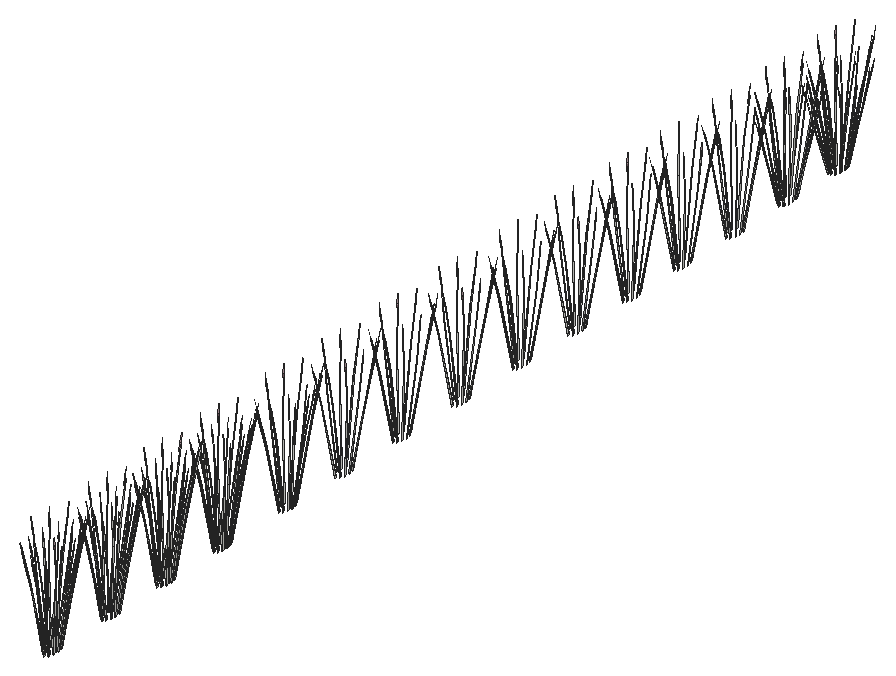
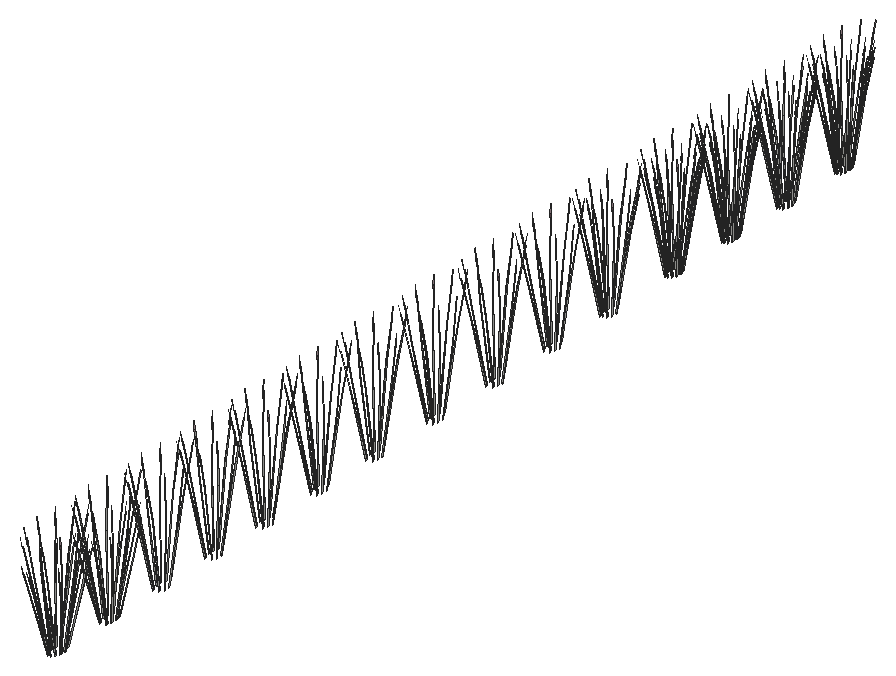
# SketchUp Ruby script. Lengths in inches.
U = 1.inch
M = Sketchup.active_model
def pt(a) = Geom::Point3d.new(a.map { |v| v * U })
def face(e, loops, mat)
  f = e.add_face(loops[0].map { |a| pt(a) })
  loops[1..].each { |l| e.add_face(l.map { |a| pt(a) }).erase! }
  f.material = f.back_material = mat if mat
  f
end
# faces: each face lists its corners as indices into pts; further lists are holes
def faces(e, pts, list, mat = nil) = list.each { |f| face(e, (f[0].is_a?(Array) ? f : [f]).map { |l| l.map { |i| pts[i] } }, mat) }
# xy, xz, yz: faces in a plane at the given z, y or x. An outline is a flat list of corners, or four numbers for a rectangle; further outlines are holes
def ring(l) = l.size == 4 ? [[l[0], l[1]], [l[2], l[1]], [l[2], l[3]], [l[0], l[3]]] : l.each_slice(2).to_a
def flat(e, list, mat, &to3) = list.each { |f| face(e, (f[0].is_a?(Array) ? f : [f]).map { |l| ring(l).map { |u, v| to3.(u, v) } }, mat) }
def xy(e, z, list, mat = nil) = flat(e, list, mat) { |x, y| [x, y, z] }
def xz(e, y, list, mat = nil) = flat(e, list, mat) { |x, z| [x, y, z] }
def yz(e, x, list, mat = nil) = flat(e, list, mat) { |y, z| [x, y, z] }
def lines(e, pts, list) = list.each { |a, b| e.add_line(pt(pts[a]), pt(pts[b])) }
# prism: a flat outline (further loops are holes) pulled along v
def prism(e, loops, v, mat = nil)
  f = face(e, loops, mat); d = Geom::Vector3d.new(v.map { |x| x * U })
  f.pushpull(f.normal.samedirection?(d) ? d.length : -d.length)
end
def box(e, o, s, mat = nil) = prism(e, [[o, [o[0] + s[0], o[1], o[2]], [o[0] + s[0], o[1] + s[1], o[2]], [o[0], o[1] + s[1], o[2]]]], [0, 0, s[2]], mat)
def at(x, y, z, deg = 0) = Geom::Transformation.translation(pt([x, y, z])) * Geom::Transformation.rotation(ORIGIN, Z_AXIS, deg.degrees)
def axes(o, x, y, z) = Geom::Transformation.new([*x, 0, *y, 0, *z, 0, *pt(o).to_a, 1])
def part(name) = M.definitions.add(name)
# library, detail: a bought-in or finely detailed component or shape, given as its bounding box
def library(name, o, s) = part(name).tap { |d| box(d.entities, o, s) }
def detail(e, o, s) = box(e.add_group.entities, o, s)
def put(e, d, t, mat = nil) = e.add_instance(d, t).tap { |i| i.material = mat if mat }
def group(e, t, mat = nil) = e.add_group.tap { |g| g.transformation = t; g.material = mat if mat }.entities
root = M.entities
M.materials.add("LightPink_Translucent").color = [144, 107, 117]
M.materials["LightPink_Translucent"].alpha = 0.75
c1 = part("blade")
p = [[2.15,0.21,22],[0,0.17,0],[0.09,0.45,0],[2.18,0.31,22],[2.29,0.31,22],[0.38,0.45,0],
  [2.48,0.24,33],[2.49,0.24,33],[2.48,0.22,33]]
faces(c1.entities,p,[[0,1,2,3],[4,5,2,3],[6,3,4,7],[8,0,3,6]])
c2 = part("seeds")
p = [[0.3,-0.1,1.38],[-0.01,-0.03,1.59],[-0.01,-0.03,0.03],[0.14,-0.07,-0.07],[0.29,-0.03,3],[0.15,0.01,3.11]]
faces(c2.entities,p,[[0,1,2,3],[1,0,4,5]],"LightPink_Translucent")
c3 = part("blade with seeds")
put(c3.entities,c1,at(0,0,0))
put(c3.entities,c2,axes([2.4,0.25,30.99],[1.5799,-0.05474,1.17369],[-0.12525,1.92788,0.29478],[-0.07173,-0.02425,1.56792]))
put(root,c3,axes([250.75,226.01,2.625],[0.01289,-0.46496,0.04667],[0.19462,0.01275,0.3674],[-0.07455,-0.04865,0.56022]))
put(root,c3,axes([252.51,225.85,2.625],[0.21034,0.02849,0.04667],[-0.00577,0.43021,0.3674],[0.02201,-0.1648,0.56022]))
put(root,c3,axes([252.58,229.75,2.625],[-0.01289,0.46496,0.04667],[-0.19462,-0.01275,0.3674],[0.07455,0.04865,0.56022]))
put(root,c3,axes([250.47,228.7,2.625],[-0.17571,-0.25715,0.04667],[0.1023,-0.3662,0.3674],[-0.05634,0.11839,0.56022]))
put(root,c3,axes([251.9375,225.18,2.625],[0.1886,-0.20781,0.04667],[0.09231,0.37894,0.3674],[-0.01821,-0.16704,0.56022]))
put(root,c3,axes([250.44,227.27,2.625],[-0.09401,-0.41691,0.04667],[0.17143,-0.20406,0.3674],[-0.07557,0.04026,0.56022]))
put(root,c3,axes([252.04,230.51,2.625],[-0.11633,0.38842,0.04667],[-0.16566,-0.22614,0.3674],[0.05356,0.12453,0.56022]))
put(root,c3,axes([250.82,229.91,2.625],[-0.21034,-0.02849,0.04667],[0.00577,-0.43021,0.3674],[-0.02201,0.1648,0.56022]))
put(root,c3,axes([251.29,240.33,2.625],[0.11633,-0.38842,0.04667],[0.16566,0.22614,0.3674],[-0.05356,-0.12453,0.56022]))
put(root,c3,axes([251.39,245.66,2.625],[-0.1886,0.20781,0.04667],[-0.09231,-0.37894,0.3674],[0.01821,0.16704,0.56022]))
put(root,c3,axes([252.86,242.14,2.625],[0.17571,0.25715,0.04667],[-0.1023,0.3662,0.3674],[0.05634,-0.11839,0.56022]))
put(root,c3,axes([252.88,243.57,2.625],[0.09401,0.41691,0.04667],[-0.17143,0.20406,0.3674],[0.07557,-0.04026,0.56022]))
put(root,c3,axes([250.75,241.09,2.625],[0.01289,-0.46496,0.04667],[0.19462,0.01275,0.3674],[-0.07455,-0.04865,0.56022]))
put(root,c3,axes([252.51,240.93,2.625],[0.21034,0.02849,0.04667],[-0.00577,0.43021,0.3674],[0.02201,-0.1648,0.56022]))
put(root,c3,axes([252.58,244.83,2.625],[-0.01289,0.46496,0.04667],[-0.19462,-0.01275,0.3674],[0.07455,0.04865,0.56022]))
put(root,c3,axes([250.47,243.78,2.625],[-0.17571,-0.25715,0.04667],[0.1023,-0.3662,0.3674],[-0.05634,0.11839,0.56022]))
put(root,c3,axes([251.9375,240.27,2.625],[0.1886,-0.20781,0.04667],[0.09231,0.37894,0.3674],[-0.01821,-0.16704,0.56022]))
put(root,c3,axes([250.44,242.36,2.625],[-0.09401,-0.41691,0.04667],[0.17143,-0.20406,0.3674],[-0.07557,0.04026,0.56022]))
put(root,c3,axes([252.04,245.6,2.625],[-0.11633,0.38842,0.04667],[-0.16566,-0.22614,0.3674],[0.05356,0.12453,0.56022]))
put(root,c3,axes([250.82,244.99,2.625],[-0.21034,-0.02849,0.04667],[0.00577,-0.43021,0.3674],[-0.02201,0.1648,0.56022]))
put(root,c3,axes([251.87,10.4375,2.63],[0.25221,0.15985,0.34839],[-0.08624,0.52553,0.28727],[-0.01516,-0.20667,0.72092]))
put(root,c3,axes([252.6,14.82,2.63],[-0.18873,0.4029,0.34839],[-0.16277,-0.42787,0.28727],[0.08855,0.07432,0.72092]))
put(root,c3,axes([252.86,13.55,2.63],[-0.07231,0.55752,0.34839],[-0.23774,-0.19064,0.28727],[0.09349,-0.0335,0.72092]))
put(root,c3,axes([250.52,14.02,2.63],[-0.06348,-0.56275,0.34839],[0.24901,-0.09767,0.28727],[-0.07339,0.13235,0.72092]))
put(root,c3,axes([250.88,15.16,2.63],[-0.18226,-0.41719,0.34839],[0.19356,-0.3598,0.28727],[-0.03362,0.19573,0.72092]))
put(root,c3,axes([252.44,11.02,2.63],[0.18226,0.41719,0.34839],[-0.19356,0.3598,0.28727],[0.03362,-0.19573,0.72092]))
put(root,c3,axes([250.46,12.63,2.63],[0.07231,-0.55752,0.34839],[0.23774,0.19064,0.28727],[-0.09349,0.0335,0.72092]))
put(root,c3,axes([252.81,12.16,2.63],[0.06348,0.56275,0.34839],[-0.24901,0.09767,0.28727],[0.07339,-0.13235,0.72092]))
put(root,c3,axes([252.08,15.62,2.63],[-0.25458,0.14032,0.34839],[-0.04418,-0.55045,0.28727],[0.05987,0.16223,0.72092]))
put(root,c3,axes([251.87,27.31,2.63],[0.25221,0.15985,0.34839],[-0.08624,0.52553,0.28727],[-0.01516,-0.20667,0.72092]))
put(root,c3,axes([252.6,31.68,2.63],[-0.18873,0.4029,0.34839],[-0.16277,-0.42787,0.28727],[0.08855,0.07432,0.72092]))
put(root,c3,axes([252.86,30.42,2.63],[-0.07231,0.55752,0.34839],[-0.23774,-0.19064,0.28727],[0.09349,-0.0335,0.72092]))
put(root,c3,axes([250.52,30.89,2.63],[-0.06348,-0.56275,0.34839],[0.24901,-0.09767,0.28727],[-0.07339,0.13235,0.72092]))
put(root,c3,axes([250.88,32.03,2.63],[-0.18226,-0.41719,0.34839],[0.19356,-0.3598,0.28727],[-0.03362,0.19573,0.72092]))
put(root,c3,axes([252.44,27.89,2.63],[0.18226,0.41719,0.34839],[-0.19356,0.3598,0.28727],[0.03362,-0.19573,0.72092]))
put(root,c3,axes([250.46,29.5,2.63],[0.07231,-0.55752,0.34839],[0.23774,0.19064,0.28727],[-0.09349,0.0335,0.72092]))
put(root,c3,axes([252.81,29.03,2.63],[0.06348,0.56275,0.34839],[-0.24901,0.09767,0.28727],[0.07339,-0.13235,0.72092]))
put(root,c3,axes([252.08,32.49,2.63],[-0.25458,0.14032,0.34839],[-0.04418,-0.55045,0.28727],[0.05987,0.16223,0.72092]))
put(root,c3,axes([251.87,43.46,2.63],[0.25221,0.15985,0.34839],[-0.08624,0.52553,0.28727],[-0.01516,-0.20667,0.72092]))
put(root,c3,axes([252.6,47.84,2.63],[-0.18873,0.4029,0.34839],[-0.16277,-0.42787,0.28727],[0.08855,0.07432,0.72092]))
put(root,c3,axes([252.86,46.57,2.63],[-0.07231,0.55752,0.34839],[-0.23774,-0.19064,0.28727],[0.09349,-0.0335,0.72092]))
put(root,c3,axes([250.52,47.04,2.63],[-0.06348,-0.56275,0.34839],[0.24901,-0.09767,0.28727],[-0.07339,0.13235,0.72092]))
put(root,c3,axes([250.88,48.18,2.63],[-0.18226,-0.41719,0.34839],[0.19356,-0.3598,0.28727],[-0.03362,0.19573,0.72092]))
put(root,c3,axes([252.44,44.04,2.63],[0.18226,0.41719,0.34839],[-0.19356,0.3598,0.28727],[0.03362,-0.19573,0.72092]))
put(root,c3,axes([250.46,45.65,2.63],[0.07231,-0.55752,0.34839],[0.23774,0.19064,0.28727],[-0.09349,0.0335,0.72092]))
put(root,c3,axes([252.81,45.18,2.63],[0.06348,0.56275,0.34839],[-0.24901,0.09767,0.28727],[0.07339,-0.13235,0.72092]))
put(root,c3,axes([252.08,48.64,2.63],[-0.25458,0.14032,0.34839],[-0.04418,-0.55045,0.28727],[0.05987,0.16223,0.72092]))
put(root,c3,axes([251.87,59.91,2.63],[0.25221,0.15985,0.34839],[-0.08624,0.52553,0.28727],[-0.01516,-0.20667,0.72092]))
put(root,c3,axes([252.6,64.29,2.63],[-0.18873,0.4029,0.34839],[-0.16277,-0.42787,0.28727],[0.08855,0.07432,0.72092]))
put(root,c3,axes([252.86,63.02,2.63],[-0.07231,0.55752,0.34839],[-0.23774,-0.19064,0.28727],[0.09349,-0.0335,0.72092]))
put(root,c3,axes([250.52,63.49,2.63],[-0.06348,-0.56275,0.34839],[0.24901,-0.09767,0.28727],[-0.07339,0.13235,0.72092]))
put(root,c3,axes([250.88,64.63,2.63],[-0.18226,-0.41719,0.34839],[0.19356,-0.3598,0.28727],[-0.03362,0.19573,0.72092]))
put(root,c3,axes([252.44,60.49,2.63],[0.18226,0.41719,0.34839],[-0.19356,0.3598,0.28727],[0.03362,-0.19573,0.72092]))
put(root,c3,axes([250.46,62.1,2.63],[0.07231,-0.55752,0.34839],[0.23774,0.19064,0.28727],[-0.09349,0.0335,0.72092]))
put(root,c3,axes([252.81,61.63,2.63],[0.06348,0.56275,0.34839],[-0.24901,0.09767,0.28727],[0.07339,-0.13235,0.72092]))
put(root,c3,axes([252.08,65.09,2.63],[-0.25458,0.14032,0.34839],[-0.04418,-0.55045,0.28727],[0.05987,0.16223,0.72092]))
put(root,c3,axes([251.87,78.93,2.63],[0.25221,0.15985,0.34839],[-0.08624,0.52553,0.28727],[-0.01516,-0.20667,0.72092]))
put(root,c3,axes([252.6,83.3125,2.63],[-0.18873,0.4029,0.34839],[-0.16277,-0.42787,0.28727],[0.08855,0.07432,0.72092]))
put(root,c3,axes([252.86,82.04,2.63],[-0.07231,0.55752,0.34839],[-0.23774,-0.19064,0.28727],[0.09349,-0.0335,0.72092]))
put(root,c3,axes([250.52,82.52,2.63],[-0.06348,-0.56275,0.34839],[0.24901,-0.09767,0.28727],[-0.07339,0.13235,0.72092]))
put(root,c3,axes([250.88,83.66,2.63],[-0.18226,-0.41719,0.34839],[0.19356,-0.3598,0.28727],[-0.03362,0.19573,0.72092]))
put(root,c3,axes([252.44,79.52,2.63],[0.18226,0.41719,0.34839],[-0.19356,0.3598,0.28727],[0.03362,-0.19573,0.72092]))
put(root,c3,axes([250.46,81.13,2.63],[0.07231,-0.55752,0.34839],[0.23774,0.19064,0.28727],[-0.09349,0.0335,0.72092]))
put(root,c3,axes([252.81,80.66,2.63],[0.06348,0.56275,0.34839],[-0.24901,0.09767,0.28727],[0.07339,-0.13235,0.72092]))
put(root,c3,axes([252.08,84.11,2.63],[-0.25458,0.14032,0.34839],[-0.04418,-0.55045,0.28727],[0.05987,0.16223,0.72092]))
put(root,c3,axes([251.87,95.51,2.63],[0.25221,0.15985,0.34839],[-0.08624,0.52553,0.28727],[-0.01516,-0.20667,0.72092]))
put(root,c3,axes([252.6,99.89,2.63],[-0.18873,0.4029,0.34839],[-0.16277,-0.42787,0.28727],[0.08855,0.07432,0.72092]))
put(root,c3,axes([252.86,98.62,2.63],[-0.07231,0.55752,0.34839],[-0.23774,-0.19064,0.28727],[0.09349,-0.0335,0.72092]))
put(root,c3,axes([250.52,99.09,2.63],[-0.06348,-0.56275,0.34839],[0.24901,-0.09767,0.28727],[-0.07339,0.13235,0.72092]))
put(root,c3,axes([250.88,100.23,2.63],[-0.18226,-0.41719,0.34839],[0.19356,-0.3598,0.28727],[-0.03362,0.19573,0.72092]))
put(root,c3,axes([252.44,96.09,2.63],[0.18226,0.41719,0.34839],[-0.19356,0.3598,0.28727],[0.03362,-0.19573,0.72092]))
put(root,c3,axes([250.46,97.71,2.63],[0.07231,-0.55752,0.34839],[0.23774,0.19064,0.28727],[-0.09349,0.0335,0.72092]))
put(root,c3,axes([252.81,97.23,2.63],[0.06348,0.56275,0.34839],[-0.24901,0.09767,0.28727],[0.07339,-0.13235,0.72092]))
put(root,c3,axes([252.08,100.69,2.63],[-0.25458,0.14032,0.34839],[-0.04418,-0.55045,0.28727],[0.05987,0.16223,0.72092]))
put(root,c3,axes([251.87,112.27,2.63],[0.25221,0.15985,0.34839],[-0.08624,0.52553,0.28727],[-0.01516,-0.20667,0.72092]))
put(root,c3,axes([252.6,116.64,2.63],[-0.18873,0.4029,0.34839],[-0.16277,-0.42787,0.28727],[0.08855,0.07432,0.72092]))
put(root,c3,axes([252.86,115.38,2.63],[-0.07231,0.55752,0.34839],[-0.23774,-0.19064,0.28727],[0.09349,-0.0335,0.72092]))
put(root,c3,axes([250.52,115.85,2.63],[-0.06348,-0.56275,0.34839],[0.24901,-0.09767,0.28727],[-0.07339,0.13235,0.72092]))
put(root,c3,axes([250.88,116.99,2.63],[-0.18226,-0.41719,0.34839],[0.19356,-0.3598,0.28727],[-0.03362,0.19573,0.72092]))
put(root,c3,axes([252.44,112.85,2.63],[0.18226,0.41719,0.34839],[-0.19356,0.3598,0.28727],[0.03362,-0.19573,0.72092]))
put(root,c3,axes([250.46,114.46,2.63],[0.07231,-0.55752,0.34839],[0.23774,0.19064,0.28727],[-0.09349,0.0335,0.72092]))
put(root,c3,axes([252.81,113.99,2.63],[0.06348,0.56275,0.34839],[-0.24901,0.09767,0.28727],[0.07339,-0.13235,0.72092]))
put(root,c3,axes([252.08,117.45,2.63],[-0.25458,0.14032,0.34839],[-0.04418,-0.55045,0.28727],[0.05987,0.16223,0.72092]))
put(root,c3,axes([251.87,129.71,2.63],[0.25221,0.15985,0.34839],[-0.08624,0.52553,0.28727],[-0.01516,-0.20667,0.72092]))
put(root,c3,axes([252.6,134.09,2.63],[-0.18873,0.4029,0.34839],[-0.16277,-0.42787,0.28727],[0.08855,0.07432,0.72092]))
put(root,c3,axes([252.86,132.82,2.63],[-0.07231,0.55752,0.34839],[-0.23774,-0.19064,0.28727],[0.09349,-0.0335,0.72092]))
put(root,c3,axes([250.52,133.3,2.63],[-0.06348,-0.56275,0.34839],[0.24901,-0.09767,0.28727],[-0.07339,0.13235,0.72092]))
put(root,c3,axes([250.88,134.43,2.63],[-0.18226,-0.41719,0.34839],[0.19356,-0.3598,0.28727],[-0.03362,0.19573,0.72092]))
put(root,c3,axes([252.44,130.3,2.63],[0.18226,0.41719,0.34839],[-0.19356,0.3598,0.28727],[0.03362,-0.19573,0.72092]))
put(root,c3,axes([250.46,131.91,2.63],[0.07231,-0.55752,0.34839],[0.23774,0.19064,0.28727],[-0.09349,0.0335,0.72092]))
put(root,c3,axes([252.81,131.43,2.63],[0.06348,0.56275,0.34839],[-0.24901,0.09767,0.28727],[0.07339,-0.13235,0.72092]))
put(root,c3,axes([252.08,134.89,2.63],[-0.25458,0.14032,0.34839],[-0.04418,-0.55045,0.28727],[0.05987,0.16223,0.72092]))
put(root,c3,axes([251.87,147.35,2.63],[0.25221,0.15985,0.34839],[-0.08624,0.52553,0.28727],[-0.01516,-0.20667,0.72092]))
put(root,c3,axes([252.6,151.73,2.63],[-0.18873,0.4029,0.34839],[-0.16277,-0.42787,0.28727],[0.08855,0.07432,0.72092]))
put(root,c3,axes([252.86,150.47,2.63],[-0.07231,0.55752,0.34839],[-0.23774,-0.19064,0.28727],[0.09349,-0.0335,0.72092]))
put(root,c3,axes([250.52,150.9375,2.63],[-0.06348,-0.56275,0.34839],[0.24901,-0.09767,0.28727],[-0.07339,0.13235,0.72092]))
put(root,c3,axes([250.88,152.08,2.63],[-0.18226,-0.41719,0.34839],[0.19356,-0.3598,0.28727],[-0.03362,0.19573,0.72092]))
put(root,c3,axes([252.44,147.9375,2.63],[0.18226,0.41719,0.34839],[-0.19356,0.3598,0.28727],[0.03362,-0.19573,0.72092]))
put(root,c3,axes([250.46,149.55,2.63],[0.07231,-0.55752,0.34839],[0.23774,0.19064,0.28727],[-0.09349,0.0335,0.72092]))
put(root,c3,axes([252.81,149.08,2.63],[0.06348,0.56275,0.34839],[-0.24901,0.09767,0.28727],[0.07339,-0.13235,0.72092]))
put(root,c3,axes([252.08,152.54,2.63],[-0.25458,0.14032,0.34839],[-0.04418,-0.55045,0.28727],[0.05987,0.16223,0.72092]))
put(root,c3,axes([251.87,163.625,2.63],[0.25221,0.15985,0.34839],[-0.08624,0.52553,0.28727],[-0.01516,-0.20667,0.72092]))
put(root,c3,axes([252.6,168,2.63],[-0.18873,0.4029,0.34839],[-0.16277,-0.42787,0.28727],[0.08855,0.07432,0.72092]))
put(root,c3,axes([252.86,166.74,2.63],[-0.07231,0.55752,0.34839],[-0.23774,-0.19064,0.28727],[0.09349,-0.0335,0.72092]))
put(root,c3,axes([250.52,167.21,2.63],[-0.06348,-0.56275,0.34839],[0.24901,-0.09767,0.28727],[-0.07339,0.13235,0.72092]))
put(root,c3,axes([250.88,168.35,2.63],[-0.18226,-0.41719,0.34839],[0.19356,-0.3598,0.28727],[-0.03362,0.19573,0.72092]))
put(root,c3,axes([252.44,164.21,2.63],[0.18226,0.41719,0.34839],[-0.19356,0.3598,0.28727],[0.03362,-0.19573,0.72092]))
put(root,c3,axes([250.46,165.82,2.63],[0.07231,-0.55752,0.34839],[0.23774,0.19064,0.28727],[-0.09349,0.0335,0.72092]))
put(root,c3,axes([252.81,165.35,2.63],[0.06348,0.56275,0.34839],[-0.24901,0.09767,0.28727],[0.07339,-0.13235,0.72092]))
put(root,c3,axes([252.08,168.81,2.63],[-0.25458,0.14032,0.34839],[-0.04418,-0.55045,0.28727],[0.05987,0.16223,0.72092]))
put(root,c3,axes([251.87,179.47,2.63],[0.25221,0.15985,0.34839],[-0.08624,0.52553,0.28727],[-0.01516,-0.20667,0.72092]))
put(root,c3,axes([252.6,183.85,2.63],[-0.18873,0.4029,0.34839],[-0.16277,-0.42787,0.28727],[0.08855,0.07432,0.72092]))
put(root,c3,axes([252.86,182.59,2.63],[-0.07231,0.55752,0.34839],[-0.23774,-0.19064,0.28727],[0.09349,-0.0335,0.72092]))
put(root,c3,axes([250.52,183.06,2.63],[-0.06348,-0.56275,0.34839],[0.24901,-0.09767,0.28727],[-0.07339,0.13235,0.72092]))
put(root,c3,axes([250.88,184.2,2.63],[-0.18226,-0.41719,0.34839],[0.19356,-0.3598,0.28727],[-0.03362,0.19573,0.72092]))
put(root,c3,axes([252.44,180.06,2.63],[0.18226,0.41719,0.34839],[-0.19356,0.3598,0.28727],[0.03362,-0.19573,0.72092]))
put(root,c3,axes([250.46,181.67,2.63],[0.07231,-0.55752,0.34839],[0.23774,0.19064,0.28727],[-0.09349,0.0335,0.72092]))
put(root,c3,axes([252.81,181.2,2.63],[0.06348,0.56275,0.34839],[-0.24901,0.09767,0.28727],[0.07339,-0.13235,0.72092]))
put(root,c3,axes([252.08,184.66,2.63],[-0.25458,0.14032,0.34839],[-0.04418,-0.55045,0.28727],[0.05987,0.16223,0.72092]))
put(root,c3,axes([251.87,194.46,2.63],[0.25221,0.15985,0.34839],[-0.08624,0.52553,0.28727],[-0.01516,-0.20667,0.72092]))
put(root,c3,axes([252.6,198.84,2.63],[-0.18873,0.4029,0.34839],[-0.16277,-0.42787,0.28727],[0.08855,0.07432,0.72092]))
put(root,c3,axes([252.86,197.57,2.63],[-0.07231,0.55752,0.34839],[-0.23774,-0.19064,0.28727],[0.09349,-0.0335,0.72092]))
put(root,c3,axes([250.52,198.05,2.63],[-0.06348,-0.56275,0.34839],[0.24901,-0.09767,0.28727],[-0.07339,0.13235,0.72092]))
put(root,c3,axes([250.88,199.18,2.63],[-0.18226,-0.41719,0.34839],[0.19356,-0.3598,0.28727],[-0.03362,0.19573,0.72092]))
put(root,c3,axes([252.44,195.05,2.63],[0.18226,0.41719,0.34839],[-0.19356,0.3598,0.28727],[0.03362,-0.19573,0.72092]))
put(root,c3,axes([250.46,196.66,2.63],[0.07231,-0.55752,0.34839],[0.23774,0.19064,0.28727],[-0.09349,0.0335,0.72092]))
put(root,c3,axes([252.81,196.18,2.63],[0.06348,0.56275,0.34839],[-0.24901,0.09767,0.28727],[0.07339,-0.13235,0.72092]))
put(root,c3,axes([252.08,199.64,2.63],[-0.25458,0.14032,0.34839],[-0.04418,-0.55045,0.28727],[0.05987,0.16223,0.72092]))
put(root,c3,axes([251.87,209.71,2.63],[0.25221,0.15985,0.34839],[-0.08624,0.52553,0.28727],[-0.01516,-0.20667,0.72092]))
put(root,c3,axes([252.6,214.09,2.63],[-0.18873,0.4029,0.34839],[-0.16277,-0.42787,0.28727],[0.08855,0.07432,0.72092]))
put(root,c3,axes([252.86,212.83,2.63],[-0.07231,0.55752,0.34839],[-0.23774,-0.19064,0.28727],[0.09349,-0.0335,0.72092]))
put(root,c3,axes([250.52,213.3,2.63],[-0.06348,-0.56275,0.34839],[0.24901,-0.09767,0.28727],[-0.07339,0.13235,0.72092]))
put(root,c3,axes([250.88,214.4375,2.63],[-0.18226,-0.41719,0.34839],[0.19356,-0.3598,0.28727],[-0.03362,0.19573,0.72092]))
put(root,c3,axes([252.44,210.3,2.63],[0.18226,0.41719,0.34839],[-0.19356,0.3598,0.28727],[0.03362,-0.19573,0.72092]))
put(root,c3,axes([250.46,211.91,2.63],[0.07231,-0.55752,0.34839],[0.23774,0.19064,0.28727],[-0.09349,0.0335,0.72092]))
put(root,c3,axes([252.81,211.4375,2.63],[0.06348,0.56275,0.34839],[-0.24901,0.09767,0.28727],[0.07339,-0.13235,0.72092]))
put(root,c3,axes([252.08,214.9,2.63],[-0.25458,0.14032,0.34839],[-0.04418,-0.55045,0.28727],[0.05987,0.16223,0.72092]))
put(root,c3,axes([251.87,225.22,2.63],[0.25221,0.15985,0.34839],[-0.08624,0.52553,0.28727],[-0.01516,-0.20667,0.72092]))
put(root,c3,axes([252.6,229.6,2.63],[-0.18873,0.4029,0.34839],[-0.16277,-0.42787,0.28727],[0.08855,0.07432,0.72092]))
put(root,c3,axes([252.86,228.34,2.63],[-0.07231,0.55752,0.34839],[-0.23774,-0.19064,0.28727],[0.09349,-0.0335,0.72092]))
put(root,c3,axes([250.52,228.81,2.63],[-0.06348,-0.56275,0.34839],[0.24901,-0.09767,0.28727],[-0.07339,0.13235,0.72092]))
put(root,c3,axes([250.88,229.95,2.63],[-0.18226,-0.41719,0.34839],[0.19356,-0.3598,0.28727],[-0.03362,0.19573,0.72092]))
put(root,c3,axes([252.44,225.81,2.63],[0.18226,0.41719,0.34839],[-0.19356,0.3598,0.28727],[0.03362,-0.19573,0.72092]))
put(root,c3,axes([250.46,227.42,2.63],[0.07231,-0.55752,0.34839],[0.23774,0.19064,0.28727],[-0.09349,0.0335,0.72092]))
put(root,c3,axes([252.81,226.95,2.63],[0.06348,0.56275,0.34839],[-0.24901,0.09767,0.28727],[0.07339,-0.13235,0.72092]))
put(root,c3,axes([252.08,230.4,2.63],[-0.25458,0.14032,0.34839],[-0.04418,-0.55045,0.28727],[0.05987,0.16223,0.72092]))
put(root,c3,axes([251.87,240.31,2.63],[0.25221,0.15985,0.34839],[-0.08624,0.52553,0.28727],[-0.01516,-0.20667,0.72092]))
put(root,c3,axes([252.6,244.69,2.63],[-0.18873,0.4029,0.34839],[-0.16277,-0.42787,0.28727],[0.08855,0.07432,0.72092]))
put(root,c3,axes([252.86,243.42,2.63],[-0.07231,0.55752,0.34839],[-0.23774,-0.19064,0.28727],[0.09349,-0.0335,0.72092]))
put(root,c3,axes([250.52,243.89,2.63],[-0.06348,-0.56275,0.34839],[0.24901,-0.09767,0.28727],[-0.07339,0.13235,0.72092]))
put(root,c3,axes([250.88,245.03,2.63],[-0.18226,-0.41719,0.34839],[0.19356,-0.3598,0.28727],[-0.03362,0.19573,0.72092]))
put(root,c3,axes([252.44,240.89,2.63],[0.18226,0.41719,0.34839],[-0.19356,0.3598,0.28727],[0.03362,-0.19573,0.72092]))
put(root,c3,axes([250.46,242.5,2.63],[0.07231,-0.55752,0.34839],[0.23774,0.19064,0.28727],[-0.09349,0.0335,0.72092]))
put(root,c3,axes([252.81,242.03,2.63],[0.06348,0.56275,0.34839],[-0.24901,0.09767,0.28727],[0.07339,-0.13235,0.72092]))
put(root,c3,axes([252.08,245.49,2.63],[-0.25458,0.14032,0.34839],[-0.04418,-0.55045,0.28727],[0.05987,0.16223,0.72092]))
put(root,c3,axes([251.46,15.36,2.86],[0.07716,-0.47021,0.25703],[0.22512,0.13715,-0.33183],[0.02064,0.18932,0.63492]))
put(root,c3,axes([251.87,10.82,2.86],[-0.07716,0.47021,0.25703],[-0.22512,-0.13715,-0.33183],[-0.02064,-0.18932,0.63492]))
put(root,c3,axes([252.45,14.62,2.86],[-0.14563,-0.38283,0.25703],[0.16629,-0.3624,-0.33183],[0.08449,0.05514,0.63492]))
put(root,c3,axes([252.69,13.54,2.86],[-0.21272,-0.17057,0.25703],[0.06204,-0.49764,-0.33183],[0.08564,-0.04563,0.63492]))
put(root,c3,axes([250.88,11.57,2.86],[0.14563,0.38283,0.25703],[-0.16629,0.3624,-0.33183],[-0.08449,-0.05514,0.63492]))
put(root,c3,axes([250.97,14.83,2.86],[0.17318,-0.32193,0.25703],[0.16394,0.36759,-0.33183],[-0.02494,0.18677,0.63492]))
put(root,c3,axes([250.67,13.83,2.86],[0.2228,-0.08739,0.25703],[0.05883,0.49954,-0.33183],[-0.06385,0.13418,0.63492]))
put(root,c3,axes([252,15.28,2.86],[-0.03953,-0.49251,0.25703],[0.22598,-0.13005,-0.33183],[0.0607,0.14114,0.63492]))
put(root,c3,axes([252.65,12.35,2.86],[-0.2228,0.08739,0.25703],[-0.05883,-0.49954,-0.33183],[0.06385,-0.13418,0.63492]))
put(root,c3,axes([250.64,12.64,2.86],[0.21272,0.17057,0.25703],[-0.06204,0.49764,-0.33183],[-0.08564,0.04563,0.63492]))
put(root,c3,axes([252.35,11.35,2.86],[-0.17318,0.32193,0.25703],[-0.16394,-0.36759,-0.33183],[0.02494,-0.18677,0.63492]))
put(root,c3,axes([251.33,10.9,2.86],[0.03953,0.49251,0.25703],[-0.22598,0.13005,-0.33183],[-0.0607,-0.14114,0.63492]))
put(root,c3,axes([251.46,32.23,2.86],[0.07716,-0.47021,0.25703],[0.22512,0.13715,-0.33183],[0.02064,0.18932,0.63492]))
put(root,c3,axes([251.87,27.69,2.86],[-0.07716,0.47021,0.25703],[-0.22512,-0.13715,-0.33183],[-0.02064,-0.18932,0.63492]))
put(root,c3,axes([252.45,31.48,2.86],[-0.14563,-0.38283,0.25703],[0.16629,-0.3624,-0.33183],[0.08449,0.05514,0.63492]))
put(root,c3,axes([252.69,30.41,2.86],[-0.21272,-0.17057,0.25703],[0.06204,-0.49764,-0.33183],[0.08564,-0.04563,0.63492]))
put(root,c3,axes([250.88,28.43,2.86],[0.14563,0.38283,0.25703],[-0.16629,0.3624,-0.33183],[-0.08449,-0.05514,0.63492]))
put(root,c3,axes([250.97,31.7,2.86],[0.17318,-0.32193,0.25703],[0.16394,0.36759,-0.33183],[-0.02494,0.18677,0.63492]))
put(root,c3,axes([250.67,30.7,2.86],[0.2228,-0.08739,0.25703],[0.05883,0.49954,-0.33183],[-0.06385,0.13418,0.63492]))
put(root,c3,axes([252,32.15,2.86],[-0.03953,-0.49251,0.25703],[0.22598,-0.13005,-0.33183],[0.0607,0.14114,0.63492]))
put(root,c3,axes([252.65,29.22,2.86],[-0.2228,0.08739,0.25703],[-0.05883,-0.49954,-0.33183],[0.06385,-0.13418,0.63492]))
put(root,c3,axes([250.64,29.51,2.86],[0.21272,0.17057,0.25703],[-0.06204,0.49764,-0.33183],[-0.08564,0.04563,0.63492]))
put(root,c3,axes([252.35,28.22,2.86],[-0.17318,0.32193,0.25703],[-0.16394,-0.36759,-0.33183],[0.02494,-0.18677,0.63492]))
put(root,c3,axes([251.33,27.77,2.86],[0.03953,0.49251,0.25703],[-0.22598,0.13005,-0.33183],[-0.0607,-0.14114,0.63492]))
put(root,c3,axes([251.46,48.38,2.86],[0.07716,-0.47021,0.25703],[0.22512,0.13715,-0.33183],[0.02064,0.18932,0.63492]))
put(root,c3,axes([251.87,43.84,2.86],[-0.07716,0.47021,0.25703],[-0.22512,-0.13715,-0.33183],[-0.02064,-0.18932,0.63492]))
put(root,c3,axes([252.45,47.64,2.86],[-0.14563,-0.38283,0.25703],[0.16629,-0.3624,-0.33183],[0.08449,0.05514,0.63492]))
put(root,c3,axes([252.69,46.5625,2.86],[-0.21272,-0.17057,0.25703],[0.06204,-0.49764,-0.33183],[0.08564,-0.04563,0.63492]))
put(root,c3,axes([250.88,44.59,2.86],[0.14563,0.38283,0.25703],[-0.16629,0.3624,-0.33183],[-0.08449,-0.05514,0.63492]))
put(root,c3,axes([250.97,47.85,2.86],[0.17318,-0.32193,0.25703],[0.16394,0.36759,-0.33183],[-0.02494,0.18677,0.63492]))
put(root,c3,axes([250.67,46.86,2.86],[0.2228,-0.08739,0.25703],[0.05883,0.49954,-0.33183],[-0.06385,0.13418,0.63492]))
put(root,c3,axes([252,48.3,2.86],[-0.03953,-0.49251,0.25703],[0.22598,-0.13005,-0.33183],[0.0607,0.14114,0.63492]))
put(root,c3,axes([252.65,45.37,2.86],[-0.2228,0.08739,0.25703],[-0.05883,-0.49954,-0.33183],[0.06385,-0.13418,0.63492]))
put(root,c3,axes([250.64,45.66,2.86],[0.21272,0.17057,0.25703],[-0.06204,0.49764,-0.33183],[-0.08564,0.04563,0.63492]))
put(root,c3,axes([252.35,44.375,2.86],[-0.17318,0.32193,0.25703],[-0.16394,-0.36759,-0.33183],[0.02494,-0.18677,0.63492]))
put(root,c3,axes([251.33,43.92,2.86],[0.03953,0.49251,0.25703],[-0.22598,0.13005,-0.33183],[-0.0607,-0.14114,0.63492]))
put(root,c3,axes([251.46,64.83,2.86],[0.07716,-0.47021,0.25703],[0.22512,0.13715,-0.33183],[0.02064,0.18932,0.63492]))
put(root,c3,axes([251.87,60.29,2.86],[-0.07716,0.47021,0.25703],[-0.22512,-0.13715,-0.33183],[-0.02064,-0.18932,0.63492]))
put(root,c3,axes([252.45,64.09,2.86],[-0.14563,-0.38283,0.25703],[0.16629,-0.3624,-0.33183],[0.08449,0.05514,0.63492]))
put(root,c3,axes([252.69,63.01,2.86],[-0.21272,-0.17057,0.25703],[0.06204,-0.49764,-0.33183],[0.08564,-0.04563,0.63492]))
put(root,c3,axes([250.88,61.04,2.86],[0.14563,0.38283,0.25703],[-0.16629,0.3624,-0.33183],[-0.08449,-0.05514,0.63492]))
put(root,c3,axes([250.97,64.3,2.86],[0.17318,-0.32193,0.25703],[0.16394,0.36759,-0.33183],[-0.02494,0.18677,0.63492]))
put(root,c3,axes([250.67,63.31,2.86],[0.2228,-0.08739,0.25703],[0.05883,0.49954,-0.33183],[-0.06385,0.13418,0.63492]))
put(root,c3,axes([252,64.75,2.86],[-0.03953,-0.49251,0.25703],[0.22598,-0.13005,-0.33183],[0.0607,0.14114,0.63492]))
put(root,c3,axes([252.65,61.82,2.86],[-0.2228,0.08739,0.25703],[-0.05883,-0.49954,-0.33183],[0.06385,-0.13418,0.63492]))
put(root,c3,axes([250.64,62.11,2.86],[0.21272,0.17057,0.25703],[-0.06204,0.49764,-0.33183],[-0.08564,0.04563,0.63492]))
put(root,c3,axes([252.35,60.82,2.86],[-0.17318,0.32193,0.25703],[-0.16394,-0.36759,-0.33183],[0.02494,-0.18677,0.63492]))
put(root,c3,axes([251.33,60.37,2.86],[0.03953,0.49251,0.25703],[-0.22598,0.13005,-0.33183],[-0.0607,-0.14114,0.63492]))
put(root,c3,axes([251.46,83.86,2.86],[0.07716,-0.47021,0.25703],[0.22512,0.13715,-0.33183],[0.02064,0.18932,0.63492]))
put(root,c3,axes([251.87,79.32,2.86],[-0.07716,0.47021,0.25703],[-0.22512,-0.13715,-0.33183],[-0.02064,-0.18932,0.63492]))
put(root,c3,axes([252.45,83.11,2.86],[-0.14563,-0.38283,0.25703],[0.16629,-0.3624,-0.33183],[0.08449,0.05514,0.63492]))
put(root,c3,axes([252.69,82.04,2.86],[-0.21272,-0.17057,0.25703],[0.06204,-0.49764,-0.33183],[0.08564,-0.04563,0.63492]))
